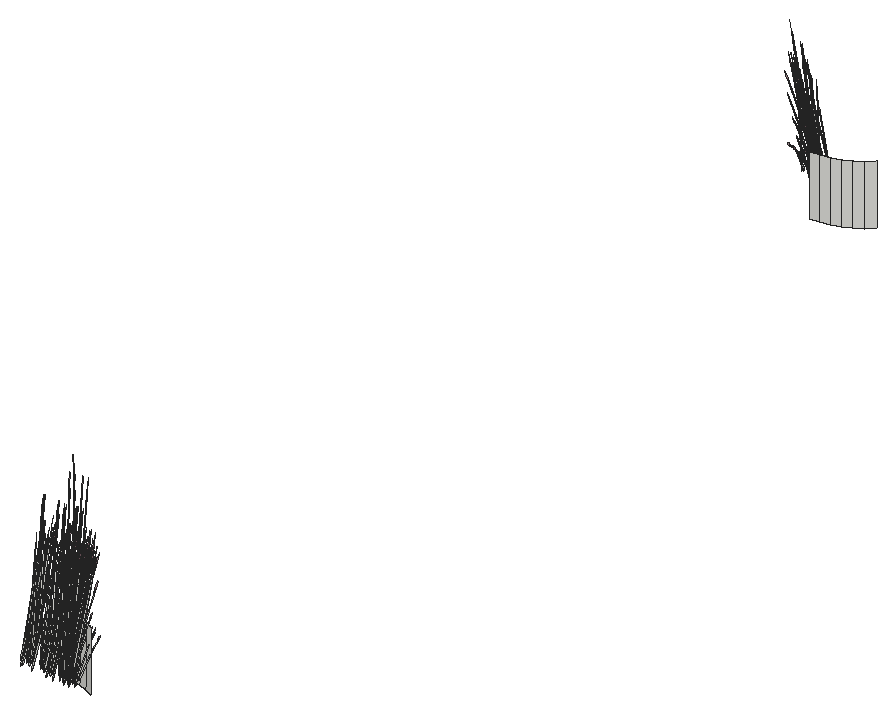
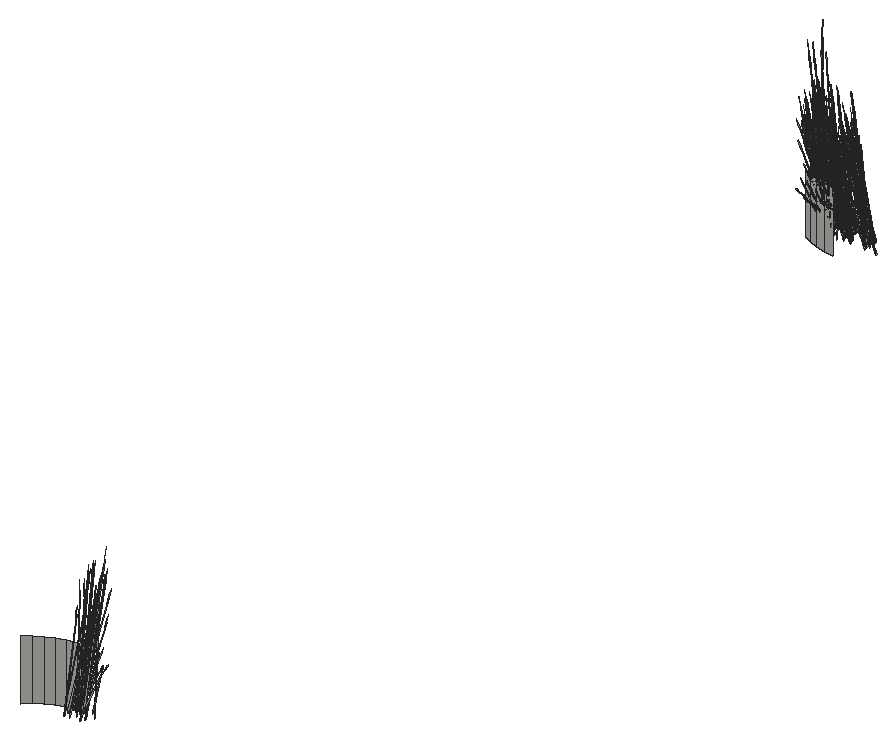
# SketchUp Ruby script. Lengths in inches.
U = 1.inch
M = Sketchup.active_model
def pt(a) = Geom::Point3d.new(a.map { |v| v * U })
def face(e, loops, mat)
  f = e.add_face(loops[0].map { |a| pt(a) })
  loops[1..].each { |l| e.add_face(l.map { |a| pt(a) }).erase! }
  f.material = f.back_material = mat if mat
  f
end
# faces: each face lists its corners as indices into pts; further lists are holes
def faces(e, pts, list, mat = nil) = list.each { |f| face(e, (f[0].is_a?(Array) ? f : [f]).map { |l| l.map { |i| pts[i] } }, mat) }
# xy, xz, yz: faces in a plane at the given z, y or x. An outline is a flat list of corners, or four numbers for a rectangle; further outlines are holes
def ring(l) = l.size == 4 ? [[l[0], l[1]], [l[2], l[1]], [l[2], l[3]], [l[0], l[3]]] : l.each_slice(2).to_a
def flat(e, list, mat, &to3) = list.each { |f| face(e, (f[0].is_a?(Array) ? f : [f]).map { |l| ring(l).map { |u, v| to3.(u, v) } }, mat) }
def xy(e, z, list, mat = nil) = flat(e, list, mat) { |x, y| [x, y, z] }
def xz(e, y, list, mat = nil) = flat(e, list, mat) { |x, z| [x, y, z] }
def yz(e, x, list, mat = nil) = flat(e, list, mat) { |y, z| [x, y, z] }
def lines(e, pts, list) = list.each { |a, b| e.add_line(pt(pts[a]), pt(pts[b])) }
# prism: a flat outline (further loops are holes) pulled along v
def prism(e, loops, v, mat = nil)
  f = face(e, loops, mat); d = Geom::Vector3d.new(v.map { |x| x * U })
  f.pushpull(f.normal.samedirection?(d) ? d.length : -d.length)
end
def box(e, o, s, mat = nil) = prism(e, [[o, [o[0] + s[0], o[1], o[2]], [o[0] + s[0], o[1] + s[1], o[2]], [o[0], o[1] + s[1], o[2]]]], [0, 0, s[2]], mat)
def at(x, y, z, deg = 0) = Geom::Transformation.translation(pt([x, y, z])) * Geom::Transformation.rotation(ORIGIN, Z_AXIS, deg.degrees)
def axes(o, x, y, z) = Geom::Transformation.new([*x, 0, *y, 0, *z, 0, *pt(o).to_a, 1])
def part(name) = M.definitions.add(name)
# library, detail: a bought-in or finely detailed component or shape, given as its bounding box
def library(name, o, s) = part(name).tap { |d| box(d.entities, o, s) }
def detail(e, o, s) = box(e.add_group.entities, o, s)
def put(e, d, t, mat = nil) = e.add_instance(d, t).tap { |i| i.material = mat if mat }
def group(e, t, mat = nil) = e.add_group.tap { |g| g.transformation = t; g.material = mat if mat }.entities
root = M.entities
M.materials.add("LightPink_Translucent").color = [144, 107, 117]
M.materials["LightPink_Translucent"].alpha = 0.75
c1 = part("blade")
p = [[2.15,0.21,22],[0,0.17,0],[0.09,0.45,0],[2.18,0.31,22],[2.29,0.31,22],[0.38,0.45,0],
  [2.48,0.24,33],[2.49,0.24,33],[2.48,0.22,33]]
faces(c1.entities,p,[[0,1,2,3],[4,5,2,3],[6,3,4,7],[8,0,3,6]])
c2 = part("seeds")
p = [[0.3,-0.1,1.38],[-0.01,-0.03,1.59],[-0.01,-0.03,0.03],[0.14,-0.07,-0.07],[0.29,-0.03,3],[0.15,0.01,3.11]]
faces(c2.entities,p,[[0,1,2,3],[1,0,4,5]],"LightPink_Translucent")
c3 = part("blade with seeds")
put(c3.entities,c1,at(0,0,0))
put(c3.entities,c2,axes([2.4,0.25,30.99],[1.5799,-0.05474,1.17369],[-0.12525,1.92788,0.29478],[-0.07173,-0.02425,1.56792]))
p = [[362.61,359.94,618],[365.07,358.73,618],[365.07,358.73,636],[362.61,359.94,636],[360.01,360.83,618],[360.01,360.83,636],
  [357.32,361.36,618],[357.32,361.36,636],[354.57,361.54,618],[354.57,361.54,636],[357.32,641.08,618],[354.57,640.9,618],
  [354.57,640.9,636],[357.32,641.08,636],[360.01,641.62,618],[360.01,641.62,636],[362.61,642.5,618],[362.61,642.5,636],
  [365.07,643.71,618],[365.07,643.71,636],[367.36,645.24,618],[367.36,645.24,636],[369.42,647.05,618],[369.42,647.05,636]]
faces(root,p,[[0,1,2,3],[4,0,3,5],[6,4,5,7],[8,6,7,9],[10,11,12,13],[14,10,13,15],[16,14,15,17],[18,16,17,19],
  [20,18,19,21],[22,20,21,23]])
put(root,c3,axes([346.59,356.8125,622.68],[0.34827,-0.11086,-0.51099],[0.06092,0.41983,-0.3958],[0.09354,0.12031,0.97773]))
put(root,c3,axes([355.35,356.44,622.73],[-0.26007,0.1585,0.0643],[-0.12729,-0.28902,0.50621],[0.02512,0.1274,0.77189]))
put(root,c3,axes([360.92,357.125,620.375],[0.22066,0.46731,0],[-0.36918,0.26061,-0.51607],[-0.08408,0.05936,1.63711]))
put(root,c3,axes([345.05,357.22,619.49],[0.02571,-0.06733,1.76342],[0.32373,-0.19829,-0.26939],[0.09815,0.10263,0.30037]))
put(root,c3,axes([354.65,356.0625,622.53],[-0.23881,0.24554,-0.35414],[-0.22606,-0.28036,0.4572],[-0.0344,0.14245,0.87481]))
put(root,c3,axes([353.83,355.99,622.72],[-0.00877,0.09229,1.74944],[0.24897,0.32105,-0.27667],[-0.06518,0.15182,0.14031]))
put(root,c3,axes([363.75,355.83,622.72],[0.04474,0.0751,1.74944],[0.36104,0.0295,-0.27667],[0.03631,0.16562,0.14031]))
put(root,c3,axes([354.62,355.78,623.4],[0.3879,0.02311,-0.13498],[-0.0106,0.43749,-0.74919],[-0.02694,0.1685,1.13838]))
put(root,c3,axes([358.7,357.49,622.71],[0.00104,-0.05646,1.77383],[0.30246,-0.2491,-0.16761],[0.10506,0.08891,0.31391]))
put(root,c3,axes([355.34,356.27,623.03],[0.34538,-0.21713,-0.1216],[0.16972,0.38536,-0.67495],[0.04557,0.16239,1.02557]))
put(root,c3,axes([360.24,357.5,622.71],[0.00104,-0.05646,1.77383],[0.30246,-0.2491,-0.16761],[0.10506,0.08891,0.31391]))
put(root,c3,axes([359.73,357.27,619.49],[0.02571,-0.06733,1.76342],[0.32373,-0.19829,-0.26939],[0.09815,0.10263,0.30037]))
put(root,c3,axes([361.27,357.28,619.49],[0.02571,-0.06733,1.76342],[0.32373,-0.19829,-0.26939],[0.09815,0.10263,0.30037]))
put(root,c3,axes([359.19,355.26,620.84],[-0.00964,-0.43909,1.41272],[0.43635,0.11382,0.59816],[-0.1032,0.24027,1.3335]))
put(root,c3,axes([359.31,355.74,620.09],[0.12941,0.42699,-0.69212],[-0.37279,0.15378,-0.18165],[0.0143,0.14459,1.52773]))
put(root,c3,axes([355.4375,356.41,623.0625],[-0.34777,-0.12192,0.53283],[0.11892,-0.40083,0.43934],[0.0209,0.15763,1.10256]))
put(root,c3,axes([352.42,355.43,621.875],[0.06572,-0.16029,1.71376],[0.27569,0.33172,0.13857],[-0.12437,0.20675,0.73262]))
put(root,c3,axes([357.38,356.84,622.73],[-0.29004,-0.02173,0.0643],[0.00795,-0.32812,0.50621],[-0.03035,0.12569,0.77189]))
put(root,c3,axes([360.73,355.28,620.84],[-0.00964,-0.43909,1.41272],[0.43635,0.11382,0.59816],[-0.1032,0.24027,1.3335]))
put(root,c3,axes([349.49,356.91,622.73],[-0.16041,0.29625,0.0643],[-0.22843,-0.17248,0.50621],[0.07385,0.09498,0.77189]))
put(root,c3,axes([360.84,355.75,620.09],[0.12941,0.42699,-0.69212],[-0.37279,0.15378,-0.18165],[0.0143,0.14459,1.52773]))
put(root,c3,axes([358.91,356.85,622.73],[-0.29004,-0.02173,0.0643],[0.00795,-0.32812,0.50621],[-0.03035,0.12569,0.77189]))
put(root,c3,axes([356.76,357.21,619.49],[0.04734,0.04659,1.76342],[0.08027,0.4317,-0.26939],[-0.10492,0.09206,0.30037]))
put(root,c3,axes([358.3,357.23,619.49],[0.04734,0.04659,1.76342],[0.08027,0.4317,-0.26939],[-0.10492,0.09206,0.30037]))
put(root,c3,axes([354.8,357.02,620.77],[-0.00913,-0.2773,1.1486],[0.22824,0.19778,0.84392],[-0.04489,0.13217,0.25299]))
put(root,c3,axes([357.47,356.87,622.73],[-0.25132,-0.3182,0.48003],[0.2669,-0.27442,0.3958],[-0.04636,0.14929,0.9933]))
put(root,c3,axes([359.23,356.96,622.68],[0.34827,-0.11086,-0.51099],[0.06092,0.41983,-0.3958],[0.09354,0.12031,0.97773]))
put(root,c3,axes([359.01,356.88,622.73],[-0.25132,-0.3182,0.48003],[0.2669,-0.27442,0.3958],[-0.04636,0.14929,0.9933]))
put(root,c3,axes([360.77,356.97,622.68],[0.34827,-0.11086,-0.51099],[0.06092,0.41983,-0.3958],[0.09354,0.12031,0.97773]))
put(root,c3,axes([349.11,357.91,623.65],[0.2439,-0.26754,-0.06488],[0.22348,0.29302,-0.29416],[0.01573,0.08303,0.97024]))
put(root,c3,axes([353.99,356,620.59],[0.00623,-0.15459,1.43002],[0.29764,-0.17268,-0.30754],[0.09188,0.18503,0.61141]))
put(root,c3,axes([349.56,356.82,622.73],[-0.35104,0.10702,0.48003],[-0.06092,-0.41983,0.3958],[0.08256,0.12373,0.9933]))
put(root,c3,axes([358.26,357.02,623.05],[0.1064,-0.35863,0.35414],[0.31043,0.1046,-0.4572],[0.02846,0.14439,0.87481]))
put(root,c3,axes([359.8,357.03,623.05],[0.1064,-0.35863,0.35414],[0.31043,0.1046,-0.4572],[0.02846,0.14439,0.87481]))
put(root,c3,axes([347.08,357.24,620.67],[-0.22633,-0.01463,1.0506],[0.14947,-0.31064,0.58006],[0.08941,0.11036,0.8241]))
put(root,c3,axes([353.19,356.72,622.73],[-0.26007,0.1585,0.0643],[-0.12729,-0.28902,0.50621],[0.02512,0.1274,0.77189]))
put(root,c3,axes([355.4,356.35,619.49],[0.05712,-0.02538,1.76342],[0.34359,0.13968,-0.26939],[0.01005,0.15742,0.30037]))
put(root,c3,axes([352.49,356.34,622.53],[-0.23881,0.24554,-0.35414],[-0.22606,-0.28036,0.4572],[-0.0344,0.14245,0.87481]))
put(root,c3,axes([351.67,356.26,622.72],[-0.00877,0.09229,1.74944],[0.24897,0.32105,-0.27667],[-0.06518,0.15182,0.14031]))
put(root,c3,axes([352.47,356.06,623.4],[0.3879,0.02311,-0.13498],[-0.0106,0.43749,-0.74919],[-0.02694,0.1685,1.13838]))
put(root,c3,axes([353.18,356.54,623.03],[0.34538,-0.21713,-0.1216],[0.16972,0.38536,-0.67495],[0.04557,0.16239,1.02557]))
put(root,c3,axes([346.42,357.16,622.73],[-0.16041,0.29625,0.0643],[-0.22843,-0.17248,0.50621],[0.07385,0.09498,0.77189]))
put(root,c3,axes([353.28,356.6875,623.0625],[-0.34777,-0.12192,0.53283],[0.11892,-0.40083,0.43934],[0.0209,0.15763,1.10256]))
put(root,c3,axes([359.71,357.38,620.67],[-0.22633,-0.01463,1.0506],[0.14947,-0.31064,0.58006],[0.08941,0.11036,0.8241]))
put(root,c3,axes([361.25,357.4,620.67],[-0.22633,-0.01463,1.0506],[0.14947,-0.31064,0.58006],[0.08941,0.11036,0.8241]))
put(root,c3,axes([352.64,357.29,620.77],[-0.00913,-0.2773,1.1486],[0.22824,0.19778,0.84392],[-0.04489,0.13217,0.25299]))
put(root,c3,axes([349.4,356.24,620.59],[0.00623,-0.15459,1.43002],[0.29764,-0.17268,-0.30754],[0.09188,0.18503,0.61141]))
put(root,c3,axes([354.89,355.95,623],[0.25266,0.31335,-0.5672],[-0.2669,0.27442,-0.43934],[-0.03844,0.15921,1.08528]))
put(root,c3,axes([346.49,357.07,622.73],[-0.35104,0.10702,0.48003],[-0.06092,-0.41983,0.3958],[0.08256,0.12373,0.9933]))
put(root,c3,axes([359.06,357.3,622.73],[-0.16041,0.29625,0.0643],[-0.22843,-0.17248,0.50621],[0.07385,0.09498,0.77189]))
put(root,c3,axes([354.61,356.42,620.82],[0.32063,-0.08258,0.06507],[0.07371,0.33271,-0.86304],[-0.02033,0.16842,0.7736]))
put(root,c3,axes([355.64,356.25,622.68],[0.34695,0.11691,-0.51099],[-0.11892,0.40083,-0.3958],[0.03181,0.16138,0.97773]))
put(root,c3,axes([360.59,357.3125,622.73],[-0.16041,0.29625,0.0643],[-0.22843,-0.17248,0.50621],[0.07385,0.09498,0.77189]))
put(root,c3,axes([348.6,356.95,622.73],[-0.26007,0.1585,0.0643],[-0.12729,-0.28902,0.50621],[0.02512,0.1274,0.77189]))
put(root,c3,axes([363.17,355.11,621.36],[0.00775,-0.24075,1.54345],[0.34877,0.12716,0.21329],[-0.03022,0.25658,0.72882]))
put(root,c3,axes([355.83,355.42,621.875],[-0.08068,-0.14973,1.71376],[0.3728,-0.12606,0.13857],[0.08426,0.23506,0.73262]))
put(root,c3,axes([347.9,356.57,622.53],[-0.23881,0.24554,-0.35414],[-0.22606,-0.28036,0.4572],[-0.0344,0.14245,0.87481]))
put(root,c3,axes([347.87,356.29,623.4],[0.3879,0.02311,-0.13498],[-0.0106,0.43749,-0.74919],[-0.02694,0.1685,1.13838]))
put(root,c3,axes([353.25,356.63,619.49],[0.05712,-0.02538,1.76342],[0.34359,0.13968,-0.26939],[0.01005,0.15742,0.30037]))
put(root,c3,axes([358.68,358.3,623.65],[0.2439,-0.26754,-0.06488],[0.22348,0.29302,-0.29416],[0.01573,0.08303,0.97024]))
put(root,c3,axes([348.59,356.78,623.03],[0.34538,-0.21713,-0.1216],[0.16972,0.38536,-0.67495],[0.04557,0.16239,1.02557]))
put(root,c3,axes([360.22,358.3125,623.65],[0.2439,-0.26754,-0.06488],[0.22348,0.29302,-0.29416],[0.01573,0.08303,0.97024]))
put(root,c3,axes([348.6875,356.92,623.0625],[-0.34777,-0.12192,0.53283],[0.11892,-0.40083,0.43934],[0.0209,0.15763,1.10256]))
put(root,c3,axes([359.125,357.22,622.73],[-0.35104,0.10702,0.48003],[-0.06092,-0.41983,0.3958],[0.08256,0.12373,0.9933]))
put(root,c3,axes([360.66,357.23,622.73],[-0.35104,0.10702,0.48003],[-0.06092,-0.41983,0.3958],[0.08256,0.12373,0.9933]))
put(root,c3,axes([348.05,357.52,620.77],[-0.00913,-0.2773,1.1486],[0.22824,0.19778,0.84392],[-0.04489,0.13217,0.25299]))
put(root,c3,axes([346.34,356.49,620.59],[0.00623,-0.15459,1.43002],[0.29764,-0.17268,-0.30754],[0.09188,0.18503,0.61141]))
put(root,c3,axes([355.48,356.5,622.53],[-0.1064,0.35863,-0.35414],[-0.31043,-0.1046,0.4572],[0.02846,0.14439,0.87481]))
put(root,c3,axes([352.73,356.22,623],[0.25266,0.31335,-0.5672],[-0.2669,0.27442,-0.43934],[-0.03844,0.15921,1.08528]))
put(root,c3,axes([357.39,356.0625,621.875],[0.06572,-0.16029,1.71376],[0.27569,0.33172,0.13857],[-0.12437,0.20675,0.73262]))
put(root,c3,axes([358.93,356.07,621.875],[0.06572,-0.16029,1.71376],[0.27569,0.33172,0.13857],[-0.12437,0.20675,0.73262]))
put(root,c3,axes([352.46,356.69,620.82],[0.32063,-0.08258,0.06507],[0.07371,0.33271,-0.86304],[-0.02033,0.16842,0.7736]))
put(root,c3,axes([353.48,356.52,622.68],[0.34695,0.11691,-0.51099],[-0.11892,0.40083,-0.3958],[0.03181,0.16138,0.97773]))
put(root,c3,axes([348.65,356.86,619.49],[0.05712,-0.02538,1.76342],[0.34359,0.13968,-0.26939],[0.01005,0.15742,0.30037]))
put(root,c3,axes([353.68,355.7,621.875],[-0.08068,-0.14973,1.71376],[0.3728,-0.12606,0.13857],[0.08426,0.23506,0.73262]))
put(root,c3,axes([358.97,356.63,620.59],[0.00623,-0.15459,1.43002],[0.29764,-0.17268,-0.30754],[0.09188,0.18503,0.61141]))
put(root,c3,axes([354.81,355.8,623.34],[-0.00918,0.43138,-0.7886],[-0.38672,-0.02897,0.09517],[-0.04081,0.18275,1.11556]))
put(root,c3,axes([360.51,356.64,620.59],[0.00623,-0.15459,1.43002],[0.29764,-0.17268,-0.30754],[0.09188,0.18503,0.61141]))
put(root,c3,axes([345.52,357.03,623.03],[0.34538,-0.21713,-0.1216],[0.16972,0.38536,-0.67495],[0.04557,0.16239,1.02557]))
put(root,c3,axes([353.8,356.9375,622.71],[0.04004,-0.02816,1.77383],[0.33095,0.18728,-0.16761],[-0.00778,0.15594,0.31391]))
put(root,c3,axes([358.17,357.35,622.73],[-0.26007,0.1585,0.0643],[-0.12729,-0.28902,0.50621],[0.02512,0.1274,0.77189]))
put(root,c3,axes([359.7,357.36,622.73],[-0.26007,0.1585,0.0643],[-0.12729,-0.28902,0.50621],[0.02512,0.1274,0.77189]))
put(root,c3,axes([357.47,356.96,622.53],[-0.23881,0.24554,-0.35414],[-0.22606,-0.28036,0.4572],[-0.0344,0.14245,0.87481]))
put(root,c3,axes([356.65,356.89,622.72],[-0.00877,0.09229,1.74944],[0.24897,0.32105,-0.27667],[-0.06518,0.15182,0.14031]))
put(root,c3,axes([348.14,356.45,623],[0.25266,0.31335,-0.5672],[-0.2669,0.27442,-0.43934],[-0.03844,0.15921,1.08528]))
put(root,c3,axes([359,356.98,622.53],[-0.23881,0.24554,-0.35414],[-0.22606,-0.28036,0.4572],[-0.0344,0.14245,0.87481]))
put(root,c3,axes([358.18,356.9,622.72],[-0.00877,0.09229,1.74944],[0.24897,0.32105,-0.27667],[-0.06518,0.15182,0.14031]))
put(root,c3,axes([357.44,356.68,623.4],[0.3879,0.02311,-0.13498],[-0.0106,0.43749,-0.74919],[-0.02694,0.1685,1.13838]))
put(root,c3,axes([358.98,356.7,623.4],[0.3879,0.02311,-0.13498],[-0.0106,0.43749,-0.74919],[-0.02694,0.1685,1.13838]))
put(root,c3,axes([358.16,357.17,623.03],[0.34538,-0.21713,-0.1216],[0.16972,0.38536,-0.67495],[0.04557,0.16239,1.02557]))
put(root,c3,axes([353.32,356.77,622.53],[-0.1064,0.35863,-0.35414],[-0.31043,-0.1046,0.4572],[0.02846,0.14439,0.87481]))
put(root,c3,axes([355.17,355.5,621.875],[-0.00864,-0.17899,1.71376],[0.37441,0.11874,0.13857],[-0.02316,0.25508,0.73262]))
put(root,c3,axes([359.7,357.18,623.03],[0.34538,-0.21713,-0.1216],[0.16972,0.38536,-0.67495],[0.04557,0.16239,1.02557]))
put(root,c3,axes([358.26,357.32,623.0625],[-0.34777,-0.12192,0.53283],[0.11892,-0.40083,0.43934],[0.0209,0.15763,1.10256]))
put(root,c3,axes([359.8,357.33,623.0625],[-0.34777,-0.12192,0.53283],[0.11892,-0.40083,0.43934],[0.0209,0.15763,1.10256]))
put(root,c3,axes([347.86,356.93,620.82],[0.32063,-0.08258,0.06507],[0.07371,0.33271,-0.86304],[-0.02033,0.16842,0.7736]))
put(root,c3,axes([348.89,356.76,622.68],[0.34695,0.11691,-0.51099],[-0.11892,0.40083,-0.3958],[0.03181,0.16138,0.97773]))
put(root,c3,axes([349.08,355.93,621.875],[-0.08068,-0.14973,1.71376],[0.3728,-0.12606,0.13857],[0.08426,0.23506,0.73262]))
put(root,c3,axes([357.62,357.92,620.77],[-0.00913,-0.2773,1.1486],[0.22824,0.19778,0.84392],[-0.04489,0.13217,0.25299]))
put(root,c3,axes([359.16,357.93,620.77],[-0.00913,-0.2773,1.1486],[0.22824,0.19778,0.84392],[-0.04489,0.13217,0.25299]))
put(root,c3,axes([352.65,356.08,623.34],[-0.00918,0.43138,-0.7886],[-0.38672,-0.02897,0.09517],[-0.04081,0.18275,1.11556]))
put(root,c3,axes([351.64,357.21,622.71],[0.04004,-0.02816,1.77383],[0.33095,0.18728,-0.16761],[-0.00778,0.15594,0.31391]))
put(root,c3,axes([355.51,356.17,622.98],[0.16845,0.3792,-0.71045],[-0.34676,0.21133,0.08574],[0.03939,0.18322,1.00501]))
put(root,c3,axes([358.22,357.26,619.49],[0.05712,-0.02538,1.76342],[0.34359,0.13968,-0.26939],[0.01005,0.15742,0.30037]))
put(root,c3,axes([359.76,357.27,619.49],[0.05712,-0.02538,1.76342],[0.34359,0.13968,-0.26939],[0.01005,0.15742,0.30037]))
put(root,c3,axes([348.73,357,622.53],[-0.1064,0.35863,-0.35414],[-0.31043,-0.1046,0.4572],[0.02846,0.14439,0.87481]))
put(root,c3,axes([353.02,355.77,621.875],[-0.00864,-0.17899,1.71376],[0.37441,0.11874,0.13857],[-0.02316,0.25508,0.73262]))
put(root,c3,axes([345.82,357.01,622.68],[0.34695,0.11691,-0.51099],[-0.11892,0.40083,-0.3958],[0.03181,0.16138,0.97773]))
put(root,c3,axes([354.53,356.77,620.59],[0.11138,-0.07357,1.43002],[0.27499,0.22183,-0.30754],[-0.08185,0.19194,0.61141]))
put(root,c3,axes([346.02,356.18,621.875],[-0.08068,-0.14973,1.71376],[0.3728,-0.12606,0.13857],[0.08426,0.23506,0.73262]))
put(root,c3,axes([348.06,356.3125,623.34],[-0.00918,0.43138,-0.7886],[-0.38672,-0.02897,0.09517],[-0.04081,0.18275,1.11556]))
put(root,c3,axes([357.71,356.85,623],[0.25266,0.31335,-0.5672],[-0.2669,0.27442,-0.43934],[-0.03844,0.15921,1.08528]))
put(root,c3,axes([355.26,357.13,622.72],[0.04474,0.0751,1.74944],[0.36104,0.0295,-0.27667],[0.03631,0.16562,0.14031]))
put(root,c3,axes([359.24,356.86,623],[0.25266,0.31335,-0.5672],[-0.2669,0.27442,-0.43934],[-0.03844,0.15921,1.08528]))
put(root,c3,axes([347.05,357.44,622.71],[0.04004,-0.02816,1.77383],[0.33095,0.18728,-0.16761],[-0.00778,0.15594,0.31391]))
put(root,c3,axes([357.43,357.32,620.82],[0.32063,-0.08258,0.06507],[0.07371,0.33271,-0.86304],[-0.02033,0.16842,0.7736]))
put(root,c3,axes([358.46,357.15,622.68],[0.34695,0.11691,-0.51099],[-0.11892,0.40083,-0.3958],[0.03181,0.16138,0.97773]))
put(root,c3,axes([358.97,357.33,620.82],[0.32063,-0.08258,0.06507],[0.07371,0.33271,-0.86304],[-0.02033,0.16842,0.7736]))
put(root,c3,axes([359.99,357.16,622.68],[0.34695,0.11691,-0.51099],[-0.11892,0.40083,-0.3958],[0.03181,0.16138,0.97773]))
put(root,c3,axes([358.65,356.33,621.875],[-0.08068,-0.14973,1.71376],[0.3728,-0.12606,0.13857],[0.08426,0.23506,0.73262]))
put(root,c3,axes([360.1875,356.34,621.875],[-0.08068,-0.14973,1.71376],[0.3728,-0.12606,0.13857],[0.08426,0.23506,0.73262]))
put(root,c3,axes([353.35,356.45,622.98],[0.16845,0.3792,-0.71045],[-0.34676,0.21133,0.08574],[0.03939,0.18322,1.00501]))
put(root,c3,axes([348.42,356.01,621.875],[-0.00864,-0.17899,1.71376],[0.37441,0.11874,0.13857],[-0.02316,0.25508,0.73262]))
put(root,c3,axes([352.38,357.04,620.59],[0.11138,-0.07357,1.43002],[0.27499,0.22183,-0.30754],[-0.08185,0.19194,0.61141]))
put(root,c3,axes([358.3,357.4,622.53],[-0.1064,0.35863,-0.35414],[-0.31043,-0.1046,0.4572],[0.02846,0.14439,0.87481]))
put(root,c3,axes([353.1,357.41,622.72],[0.04474,0.0751,1.74944],[0.36104,0.0295,-0.27667],[0.03631,0.16562,0.14031]))
put(root,c3,axes([359.83,357.41,622.53],[-0.1064,0.35863,-0.35414],[-0.31043,-0.1046,0.4572],[0.02846,0.14439,0.87481]))
put(root,c3,axes([348.76,356.68,622.98],[0.16845,0.3792,-0.71045],[-0.34676,0.21133,0.08574],[0.03939,0.18322,1.00501]))
put(root,c3,axes([357.63,356.71,623.34],[-0.00918,0.43138,-0.7886],[-0.38672,-0.02897,0.09517],[-0.04081,0.18275,1.11556]))
put(root,c3,axes([359.16,356.72,623.34],[-0.00918,0.43138,-0.7886],[-0.38672,-0.02897,0.09517],[-0.04081,0.18275,1.11556]))
put(root,c3,axes([356.62,357.84,622.71],[0.04004,-0.02816,1.77383],[0.33095,0.18728,-0.16761],[-0.00778,0.15594,0.31391]))
put(root,c3,axes([358.15,357.85,622.71],[0.04004,-0.02816,1.77383],[0.33095,0.18728,-0.16761],[-0.00778,0.15594,0.31391]))
put(root,c3,axes([354.68,356.41,621.36],[0.00775,-0.24075,1.54345],[0.34877,0.12716,0.21329],[-0.03022,0.25658,0.72882]))
put(root,c3,axes([348.51,357.64,622.72],[0.04474,0.0751,1.74944],[0.36104,0.0295,-0.27667],[0.03631,0.16562,0.14031]))
put(root,c3,axes([357.99,356.4,621.875],[-0.00864,-0.17899,1.71376],[0.37441,0.11874,0.13857],[-0.02316,0.25508,0.73262]))
put(root,c3,axes([359.53,356.41,621.875],[-0.00864,-0.17899,1.71376],[0.37441,0.11874,0.13857],[-0.02316,0.25508,0.73262]))
put(root,c3,axes([358.33,357.08,622.98],[0.16845,0.3792,-0.71045],[-0.34676,0.21133,0.08574],[0.03939,0.18322,1.00501]))
put(root,c3,axes([359.87,357.09,622.98],[0.16845,0.3792,-0.71045],[-0.34676,0.21133,0.08574],[0.03939,0.18322,1.00501]))
put(root,c3,axes([352.52,356.68,621.36],[0.00775,-0.24075,1.54345],[0.34877,0.12716,0.21329],[-0.03022,0.25658,0.72882]))
put(root,c3,axes([357.35,357.67,620.59],[0.11138,-0.07357,1.43002],[0.27499,0.22183,-0.30754],[-0.08185,0.19194,0.61141]))
put(root,c3,axes([358.89,357.69,620.59],[0.11138,-0.07357,1.43002],[0.27499,0.22183,-0.30754],[-0.08185,0.19194,0.61141]))
put(root,c3,axes([358.08,358.03,622.72],[0.04474,0.0751,1.74944],[0.36104,0.0295,-0.27667],[0.03631,0.16562,0.14031]))
put(root,c3,axes([359.61,358.05,622.72],[0.04474,0.0751,1.74944],[0.36104,0.0295,-0.27667],[0.03631,0.16562,0.14031]))
put(root,c3,axes([347.93,356.92,621.36],[0.00775,-0.24075,1.54345],[0.34877,0.12716,0.21329],[-0.03022,0.25658,0.72882]))
put(root,c3,axes([357.5,357.3125,621.36],[0.00775,-0.24075,1.54345],[0.34877,0.12716,0.21329],[-0.03022,0.25658,0.72882]))
put(root,c3,axes([359.03,357.33,621.36],[0.00775,-0.24075,1.54345],[0.34877,0.12716,0.21329],[-0.03022,0.25658,0.72882]))
put(root,c3,axes([348.63,648.61,624.94],[-0.05398,-0.06539,1.74944],[-0.36026,0.04145,-0.27667],[-0.0575,-0.15639,0.14031]))
put(root,c3,axes([349.47,649.38,622.82],[-0.10032,0.0944,1.43002],[-0.30046,-0.16522,-0.30754],[0.05569,-0.20547,0.61141]))
put(root,c3,axes([349.01,649.71,625.21],[-0.16845,-0.3792,-0.71045],[0.34676,-0.21133,0.08574],[-0.03939,-0.18322,1.00501]))
put(root,c3,axes([349.21,649.84,623.57],[0.08068,0.14973,1.71376],[-0.3728,0.12606,0.13857],[-0.08426,-0.23506,0.73262]))
put(root,c3,axes([349.82,648.84,624.41],[-0.05398,-0.06539,1.74944],[-0.36026,0.04145,-0.27667],[-0.0575,-0.15639,0.14031]))
put(root,c3,axes([348.72,648.87,621.72],[-0.0592,0.0168,1.76342],[-0.32738,-0.18913,-0.26939],[0.00549,-0.15776,0.30037]))
put(root,c3,axes([350.66,649.62,622.28],[-0.10032,0.0944,1.43002],[-0.30046,-0.16522,-0.30754],[0.05569,-0.20547,0.61141]))
put(root,c3,axes([350.2,649.95,624.67],[-0.16845,-0.3792,-0.71045],[0.34676,-0.21133,0.08574],[-0.03939,-0.18322,1.00501]))
put(root,c3,axes([346.13,649.23,624.44],[-0.00341,-0.09282,1.74944],[-0.28775,-0.26825,-0.27667],[0.04449,-0.16261,0.14031]))
put(root,c3,axes([345.16,649.68,623.6],[-0.06572,0.16029,1.71376],[-0.27569,-0.33172,0.13857],[0.12437,-0.20675,0.73262]))
put(root,c3,axes([349.11,649.44,622.28],[-0.02137,0.15256,1.43002],[-0.31245,0.12771,-0.30754],[-0.07303,-0.19719,0.61141]))
put(root,c3,axes([349.71,650.08,625.21],[0.00918,-0.43138,-0.71045],[0.38672,0.02897,0.08574],[0.04081,-0.18275,1.00501]))
put(root,c3,axes([349.91,649.11,621.18],[-0.0592,0.0168,1.76342],[-0.32738,-0.18913,-0.26939],[0.00549,-0.15776,0.30037]))
put(root,c3,axes([350.25,649.41,624.94],[-0.00341,-0.09282,1.74944],[-0.28775,-0.26825,-0.27667],[0.04449,-0.16261,0.14031]))
put(root,c3,axes([349.04,649.39,624.75],[0.1064,-0.35863,-0.35414],[0.31043,0.1046,0.4572],[-0.02846,-0.14439,0.87481]))
put(root,c3,axes([349.27,649.86,624.1],[-0.06572,0.16029,1.71376],[-0.27569,-0.33172,0.13857],[0.12437,-0.20675,0.73262]))
put(root,c3,axes([350.17,649.07,624.93],[-0.03584,0.03562,1.77383],[-0.35118,-0.12018,-0.16761],[-0.01271,-0.15545,0.31391]))
put(root,c3,axes([350.9,650.32,624.67],[0.00918,-0.43138,-0.71045],[0.38672,0.02897,0.08574],[0.04081,-0.18275,1.00501]))
put(root,c3,axes([348.88,649.63,624.91],[-0.34695,-0.11691,-0.51099],[0.11892,-0.40083,-0.3958],[-0.03181,-0.16138,0.97773]))
put(root,c3,axes([349.1,648.63,622.99],[0.04528,0.27194,1.1486],[-0.25117,-0.15062,0.84392],[0.02703,-0.13924,0.25299]))
put(root,c3,axes([351.44,649.64,624.41],[-0.00341,-0.09282,1.74944],[-0.28775,-0.26825,-0.27667],[0.04449,-0.16261,0.14031]))
put(root,c3,axes([350.23,649.625,624.22],[0.1064,-0.35863,-0.35414],[0.31043,0.1046,0.4572],[-0.02846,-0.14439,0.87481]))
put(root,c3,axes([350.47,650.1,623.57],[-0.06572,0.16029,1.71376],[-0.27569,-0.33172,0.13857],[0.12437,-0.20675,0.73262]))
put(root,c3,axes([351.37,649.3125,624.4],[-0.03584,0.03562,1.77383],[-0.35118,-0.12018,-0.16761],[-0.01271,-0.15545,0.31391]))
put(root,c3,axes([349.63,649.9375,624.91],[-0.25266,-0.31335,-0.51099],[0.2669,-0.27442,-0.3958],[0.03844,-0.15921,0.97773]))
put(root,c3,axes([352.22,650.65,623.01],[0.08068,0.14973,1.71376],[-0.3728,0.12606,0.13857],[-0.08426,-0.23506,0.73262]))
put(root,c3,axes([350.08,649.87,624.37],[-0.34695,-0.11691,-0.51099],[0.11892,-0.40083,-0.3958],[-0.03181,-0.16138,0.97773]))
put(root,c3,axes([350.29,648.87,622.46],[0.04528,0.27194,1.1486],[-0.25117,-0.15062,0.84392],[0.02703,-0.13924,0.25299]))
put(root,c3,axes([352.84,649.66,623.85],[-0.05398,-0.06539,1.74944],[-0.36026,0.04145,-0.27667],[-0.0575,-0.15639,0.14031]))
put(root,c3,axes([350.82,650.17,624.37],[-0.25266,-0.31335,-0.51099],[0.2669,-0.27442,-0.3958],[0.03844,-0.15921,0.97773]))
put(root,c3,axes([348.1875,649.38,625.32],[0.39316,-0.11987,0.53763],[0.06823,0.47021,0.4433],[-0.09247,-0.13858,1.11249]))
put(root,c3,axes([353.68,650.43,621.73],[-0.10032,0.0944,1.43002],[-0.30046,-0.16522,-0.30754],[0.05569,-0.20547,0.61141]))
put(root,c3,axes([353.22,650.76,624.12],[-0.16845,-0.3792,-0.71045],[0.34676,-0.21133,0.08574],[-0.03939,-0.18322,1.00501]))
put(root,c3,axes([349.45,648.63,624.4],[-0.00658,0.0559,1.77383],[-0.32474,0.20287,-0.16761],[-0.09556,-0.1037,0.31391]))
put(root,c3,axes([349.08,649.47,624.96],[0.34777,0.12192,0.48003],[-0.11892,0.40083,0.3958],[-0.0209,-0.15763,0.9933]))
put(root,c3,axes([349.18,649.61,625.26],[-0.34538,0.21713,-0.1216],[-0.16972,-0.38536,-0.67495],[-0.04557,-0.16239,1.02557]))
put(root,c3,axes([349.9,650.1,625.26],[-0.3879,-0.02311,-0.1216],[0.0106,-0.43749,-0.67495],[0.02694,-0.1685,1.02557]))
put(root,c3,axes([352.12,650.25,621.73],[-0.02137,0.15256,1.43002],[-0.31245,0.12771,-0.30754],[-0.07303,-0.19719,0.61141]))
put(root,c3,axes([349.87,649.82,624.75],[0.23881,-0.24554,-0.35414],[0.22606,0.28036,0.4572],[0.0344,-0.14245,0.87481]))
